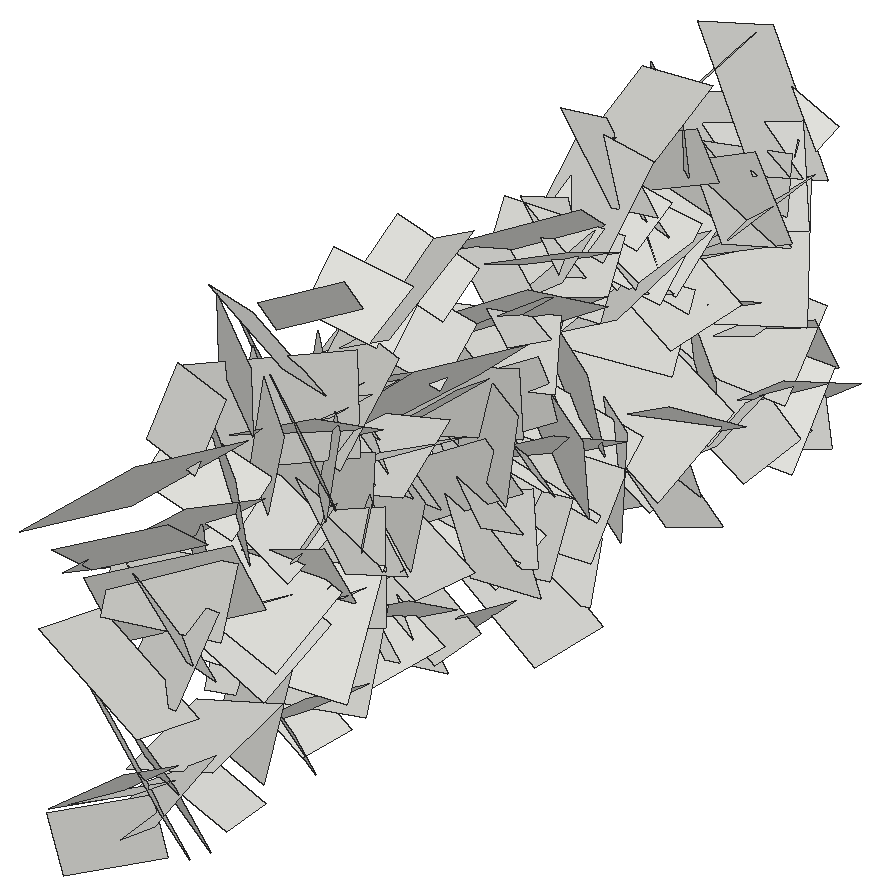
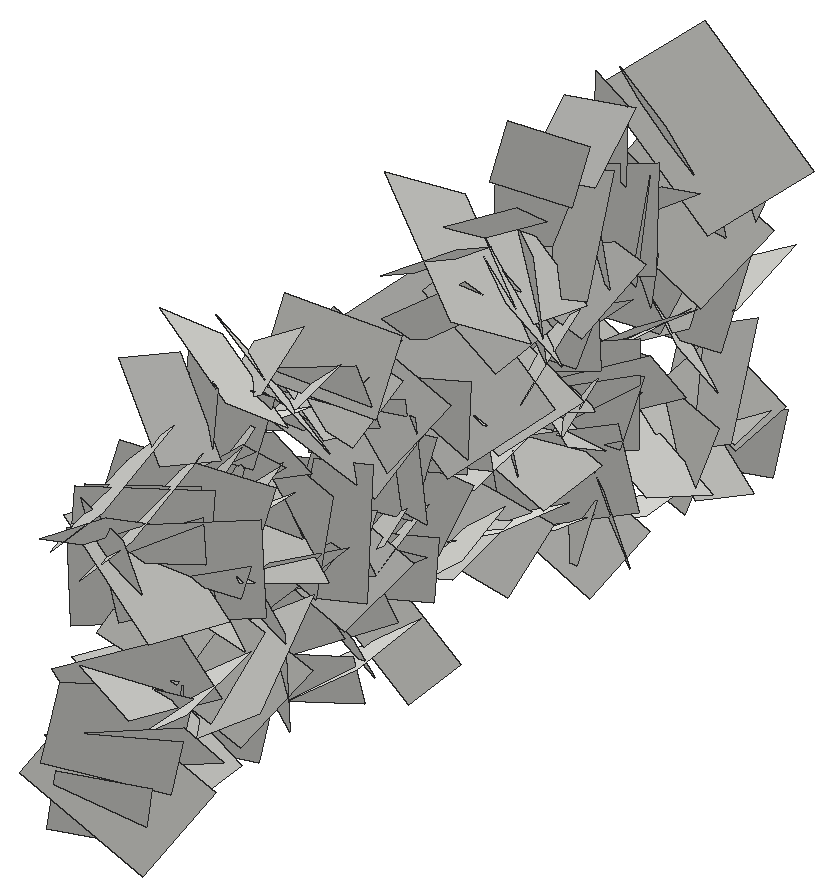
# SketchUp Ruby script. Lengths in inches.
U = 1.inch
M = Sketchup.active_model
def pt(a) = Geom::Point3d.new(a.map { |v| v * U })
def face(e, loops, mat)
  f = e.add_face(loops[0].map { |a| pt(a) })
  loops[1..].each { |l| e.add_face(l.map { |a| pt(a) }).erase! }
  f.material = f.back_material = mat if mat
  f
end
# faces: each face lists its corners as indices into pts; further lists are holes
def faces(e, pts, list, mat = nil) = list.each { |f| face(e, (f[0].is_a?(Array) ? f : [f]).map { |l| l.map { |i| pts[i] } }, mat) }
# xy, xz, yz: faces in a plane at the given z, y or x. An outline is a flat list of corners, or four numbers for a rectangle; further outlines are holes
def ring(l) = l.size == 4 ? [[l[0], l[1]], [l[2], l[1]], [l[2], l[3]], [l[0], l[3]]] : l.each_slice(2).to_a
def flat(e, list, mat, &to3) = list.each { |f| face(e, (f[0].is_a?(Array) ? f : [f]).map { |l| ring(l).map { |u, v| to3.(u, v) } }, mat) }
def xy(e, z, list, mat = nil) = flat(e, list, mat) { |x, y| [x, y, z] }
def xz(e, y, list, mat = nil) = flat(e, list, mat) { |x, z| [x, y, z] }
def yz(e, x, list, mat = nil) = flat(e, list, mat) { |y, z| [x, y, z] }
def lines(e, pts, list) = list.each { |a, b| e.add_line(pt(pts[a]), pt(pts[b])) }
# prism: a flat outline (further loops are holes) pulled along v
def prism(e, loops, v, mat = nil)
  f = face(e, loops, mat); d = Geom::Vector3d.new(v.map { |x| x * U })
  f.pushpull(f.normal.samedirection?(d) ? d.length : -d.length)
end
def box(e, o, s, mat = nil) = prism(e, [[o, [o[0] + s[0], o[1], o[2]], [o[0] + s[0], o[1] + s[1], o[2]], [o[0], o[1] + s[1], o[2]]]], [0, 0, s[2]], mat)
def at(x, y, z, deg = 0) = Geom::Transformation.translation(pt([x, y, z])) * Geom::Transformation.rotation(ORIGIN, Z_AXIS, deg.degrees)
def axes(o, x, y, z) = Geom::Transformation.new([*x, 0, *y, 0, *z, 0, *pt(o).to_a, 1])
def part(name) = M.definitions.add(name)
# library, detail: a bought-in or finely detailed component or shape, given as its bounding box
def library(name, o, s) = part(name).tap { |d| box(d.entities, o, s) }
def detail(e, o, s) = box(e.add_group.entities, o, s)
def put(e, d, t, mat = nil) = e.add_instance(d, t).tap { |i| i.material = mat if mat }
def group(e, t, mat = nil) = e.add_group.tap { |g| g.transformation = t; g.material = mat if mat }.entities
root = M.entities
c1 = part("Component\#6")
p = [[0.01,0,0],[0,3.24,4.54],[4.32,3.24,4.54],[4.33,0,0]]
faces(c1.entities,p,[[0,1,2,3]])
put(root,c1,axes([400.91,170.73,19.61],[-0.06378,-0.15247,0.68566],[-0.07422,0.68605,0.14641],[0.74085,0.05561,0.0737]))
put(root,c1,axes([400.91,173.11,21.9],[-0.05319,-0.68826,0.19248],[-0.04456,0.19546,0.68797],[0.75624,-0.03689,0.05408]))
put(root,c1,axes([400.91,173.15,22.23],[0.01199,-0.5915,0.12784],[0.10227,0.12799,0.58366],[0.63327,-0.00947,-0.09668]))
put(root,c1,axes([404.88,174.01,26.46],[0.07872,-0.97306,0.24072],[-0.0738,0.23579,0.97461],[-1.05998,-0.08868,-0.04998]))
put(root,c1,axes([404.88,172.13,35.78],[-0.07615,0.65901,-0.5201],[-0.04859,-0.52431,-0.658],[-0.88857,-0.02781,0.08055]))
put(root,c1,axes([404.88,173.5,20.5],[0.29119,-0.77592,0.90535],[-0.00734,0.92801,0.79744],[-1.26387,-0.18415,0.20396]))
put(root,c1,axes([404.88,170.16,39.2],[0.24703,1.2789,-0.21613],[0.13589,-0.24123,-1.28918],[-1.36812,0.20696,-0.16707]))
put(root,c1,axes([404.88,171.36,22.89],[-0.02535,0.88672,0.32576],[0.06435,0.32663,-0.88464],[-0.99927,-0.00146,-0.06523]))
put(root,c1,axes([404.88,173.31,35.98],[0.01252,1.07454,-0.37217],[0.12805,-0.37127,-1.06811],[-1.19858,-0.02844,-0.11799]))
put(root,c1,axes([404.88,176.41,32.2],[-0.11408,-0.0942,-0.79779],[-0.0272,-0.8041,0.09841],[-0.85109,0.03832,0.10379]))
put(root,c1,axes([404.88,172.625,27.43],[0.01975,0.58315,0.74345],[-0.01761,0.74368,-0.58292],[-1.00141,-0.00157,0.02491]))
put(root,c1,axes([404.88,174.78,20.26],[-0.10048,-0.39109,0.79293],[-0.10042,0.79738,0.38196],[-0.93179,-0.04376,-0.12667]))
put(root,c1,axes([400.91,174.375,32.02],[-0.18574,0.64681,-0.5499],[-0.00393,-0.56207,-0.65994],[0.8999,0.13105,-0.11638]))
put(root,c1,axes([404.88,176.05,33.17],[-0.01986,0.50916,-0.88553],[0.06176,-0.8837,-0.50934],[-1.08099,-0.05984,-0.01283]))
put(root,c1,axes([400.91,177.7,39.03],[-0.08239,-0.33737,-0.64844],[0.10668,-0.65083,0.32654],[0.76743,0.05425,-0.11501]))
put(root,c1,axes([400.91,178.15,33.23],[0.08938,-0.00525,-0.60269],[-0.06829,-0.60515,-0.00374],[0.63521,-0.06432,0.0844]))
put(root,c1,axes([404.88,174.9,23.69],[0.06803,0.90477,0.33383],[-0.16872,0.33992,-0.89067],[-1.00823,0.00417,0.17157]))
put(root,c1,axes([400.91,175.43,34.87],[-0.0411,0.62613,0.35799],[-0.03637,0.3565,-0.62724],[0.76365,0.05068,-0.01061]))
put(root,c1,axes([400.91,176.44,21.6],[-0.04345,0.60879,-0.00304],[0.10651,0.00376,-0.60183],[0.63647,0.04093,0.10051]))
put(root,c1,axes([404.88,177.13,31.79],[0.078,-0.30439,1.03044],[0.07955,1.03178,0.29943],[-1.13614,0.05135,0.09171]))
put(root,c1,axes([404.88,182.1,27.04],[0.18817,-1.1788,-0.21223],[0.10509,-0.19936,1.19019],[-1.26526,-0.19187,0.06729]))
put(root,c1,axes([400.91,180.11,41],[-0.0874,0.13713,-0.78202],[-0.02965,-0.78624,-0.13492],[0.84107,-0.01347,-0.08602]))
put(root,c1,axes([400.91,180.68,27.18],[-0.06604,-0.60003,0.10008],[0.10227,0.08959,0.59716],[0.63666,-0.07663,-0.08554]))
put(root,c1,axes([404.88,182.77,28.15],[0.11013,-1.0722,-0.31704],[0.03816,-0.31503,1.07721],[-1.18456,-0.10983,0.00522]))
put(root,c1,axes([404.88,178.01,21.81],[-0.00864,0.40014,0.99077],[0.02339,0.99065,-0.39991],[-1.13239,0.01741,-0.01582]))
put(root,c1,axes([400.91,182.27,37.76],[-0.22679,0.05489,-0.89691],[-0.06736,-0.9206,-0.04118],[0.95012,-0.05216,-0.217]))
put(root,c1,axes([404.88,181.8125,37.17],[0.0246,-0.63961,0.56311],[-0.17949,0.54862,0.63013],[-0.88529,-0.129,-0.11211]))
put(root,c1,axes([404.88,185.38,28.27],[0.28552,-0.8956,-0.93898],[0.07116,-0.9481,0.92355],[-1.37362,-0.23528,-0.14733]))
put(root,c1,axes([404.88,183.67,38.38],[-0.04708,0.10578,-1.15378],[0.2342,-1.13267,-0.11235],[-1.2056,-0.22416,0.02323]))
put(root,c1,axes([400.91,179.78,31.84],[-0.01485,0.68647,0.23212],[-0.1576,0.2245,-0.67291],[0.75179,0.06062,-0.13648]))
put(root,c1,axes([404.88,181.64,30.57],[-0.02444,0.48831,-0.77146],[-0.19424,-0.75848,-0.47462],[-0.9481,0.1428,0.11713]))
put(root,c1,axes([400.91,183.98,26.9],[-0.15473,-0.64925,-0.29626],[0.07231,-0.3137,0.65387],[0.75301,-0.10329,-0.12366]))
put(root,c1,axes([400.91,181.88,29.24],[0.0732,0.47057,-0.46808],[-0.06498,-0.46407,-0.47558],[0.70054,-0.09222,0.00479]))
put(root,c1,axes([404.88,180.55,24.45],[-0.04702,0.95483,-0.28451],[0.08229,-0.28062,-0.95386],[-1.05288,-0.06457,-0.06184]))
put(root,c1,axes([400.91,182.11,23.57],[-0.01533,0.32032,-0.55846],[0.07998,-0.55391,-0.31966],[0.67773,0.07262,0.02509]))
put(root,c1,axes([404.88,182.41,31.86],[0.21699,-0.67676,1.03332],[-0.0082,1.04669,0.68705],[-1.3093,-0.11872,0.16695]))
put(root,c1,axes([404.88,181.12,36.49],[0.0887,0.85058,-0.45713],[-0.14057,-0.44437,-0.85112],[-1.01388,0.13603,0.07801]))
put(root,c1,axes([400.91,184.65,28.76],[0.04824,-0.62434,-0.28052],[-0.09786,-0.28417,0.61748],[0.7189,0.00321,0.10288]))
put(root,c1,axes([404.88,185.4,30.76],[0.02152,-0.00963,-1.2106],[0.23963,-1.18945,0.01326],[-1.26071,-0.22625,-0.01814]))
put(root,c1,axes([400.91,181.75,22.9],[0.07496,0.59984,0.04506],[0.05269,0.03939,-0.60235],[0.63545,-0.07402,0.04463]))
put(root,c1,axes([404.88,185.55,26.35],[-0.05433,-0.24183,-1.04679],[0.06418,-1.04696,0.23891],[-1.13701,-0.04754,0.0635]))
put(root,c1,axes([404.88,184.8,33.37],[-0.19651,0.19461,-0.78555],[0.01158,-0.80522,-0.20206],[-0.85778,-0.05545,0.17724]))
put(root,c1,axes([400.91,183.74,37.84],[0.08456,-0.37494,0.46177],[-0.03825,0.46199,0.38136],[0.62935,0.07846,-0.03886]))
put(root,c1,axes([400.91,183.4375,30.23],[-0.10865,-0.24445,0.66529],[0.00738,0.67183,0.24793],[0.75127,-0.04195,0.09378]))
put(root,c1,axes([400.91,186.27,36.66],[-0.23271,0.08267,-1.0169],[-0.17131,-1.02986,-0.04883],[1.06781,-0.14721,-0.22945]))
put(root,c1,axes([404.88,182.86,27.86],[-0.00866,0.87216,-0.09866],[-0.12421,-0.09886,-0.86427],[-0.92206,0.00513,0.11735]))
put(root,c1,axes([400.91,186.9,33.68],[-0.12726,-0.80704,-0.07778],[0.05104,-0.08559,0.81372],[0.85791,-0.11462,-0.05995]))
put(root,c1,axes([404.88,186.8,27.07],[0.11611,-1.02809,0.5245],[0.14127,0.5346,1.02006],[-1.21522,-0.03608,0.16869]))
put(root,c1,axes([404.88,182.62,33.52],[0.16113,0.63843,0.91206],[0.00988,0.91976,-0.64538],[-1.18006,0.09488,0.11913]))
put(root,c1,axes([400.91,188.3,31.13],[-0.1103,-0.11339,-0.88165],[-0.13763,-0.87621,0.12802],[0.93214,-0.14279,-0.08543]))
put(root,c1,axes([400.91,188.62,32.29],[-0.0866,-0.74743,0.19758],[-0.06186,0.20408,0.74787],[0.81715,-0.06376,0.07755]))
put(root,c1,axes([400.91,185.35,37.93],[-0.06077,0.5182,0.40006],[0.00909,0.40215,-0.51968],[0.69387,0.04012,0.04185]))
put(root,c1,axes([404.88,189.07,22.99],[-0.09993,-0.91741,-0.05408],[-0.10319,-0.04408,0.91762],[-0.96866,0.09934,-0.09218]))
put(root,c1,axes([404.88,184.85,32.98],[0.15473,1.07562,-0.16592],[-0.16403,-0.14519,-1.07739],[-1.14193,0.1666,0.13228]))
put(root,c1,axes([404.88,186.85,26],[-0.04759,0.74401,-0.43208],[-0.09551,-0.43435,-0.73856],[-0.90698,0.0067,0.10045]))
put(root,c1,axes([404.88,186.48,30.64],[-0.03295,0.70699,0.47041],[-0.18441,0.45544,-0.69599],[-0.88105,-0.12176,0.12808]))
put(root,c1,axes([400.91,189.49,31],[-0.19159,0.03614,-0.77666],[0.1449,-0.78347,-0.06827],[0.81131,0.14846,-0.17121]))
put(root,c1,axes([404.88,189.24,21.76],[-0.15995,-0.688,0.38857],[0.02017,0.39231,0.70202],[-0.83731,0.14088,-0.05731]))
put(root,c1,axes([404.88,190.89,25.45],[0.07637,-0.93381,0.1535],[-0.06656,0.14888,0.93522],[-1.00091,-0.08115,-0.05048]))
put(root,c1,axes([400.91,188.48,31.6],[0.00806,0.51701,-0.38199],[0.06142,-0.38101,-0.51453],[0.67861,0.02834,0.0511]))
put(root,c1,axes([404.88,185.63,37.94],[0.10296,1.07287,0.66666],[0.13207,0.65722,-1.07584],[-1.33238,0.14805,-0.05512]))
put(root,c1,axes([404.88,187.18,35.87],[0.21905,1.32848,-0.23139],[0.18572,-0.25856,-1.32798],[-1.41727,0.17144,-0.20979]))
put(root,c1,axes([400.91,188.01,25.87],[-0.18323,0.88768,-0.1275],[-0.06793,-0.14175,-0.89995],[0.94816,0.16139,-0.08912]))
put(root,c1,axes([400.91,188.41,35.3125],[0.03073,0.48255,0.4704],[-0.10717,0.46862,-0.47449],[0.70624,0.05011,-0.09248]))
put(root,c1,axes([400.91,188.93,38.32],[-0.06934,0.59373,0.25],[0.00198,0.25145,-0.59671],[0.68287,0.05956,0.02711]))
put(root,c1,axes([400.91,193.29,29.97],[0.02765,-0.60791,0.13872],[-0.08921,0.13414,0.60366],[0.6549,0.04394,0.07638]))
put(root,c1,axes([400.91,192.39,25.48],[-0.15082,-0.34829,0.66058],[-0.01541,0.67363,0.35204],[0.79143,-0.05326,0.13274]))
put(root,c1,axes([404.88,193.58,33.2],[-0.1306,0.22319,-0.86205],[-0.05382,-0.87061,-0.21815],[-0.94237,0.01879,0.13193]))
put(root,c1,axes([400.91,194.26,19.42],[-0.05867,-0.70774,0.13488],[-0.12622,0.14241,0.69835],[0.75321,-0.03127,0.12754]))
put(root,c1,axes([404.88,192.76,27.5],[0.21382,-0.08753,1.03604],[-0.20559,1.03367,0.1251],[-1.08277,-0.21355,0.18084]))
put(root,c1,axes([400.91,192.62,23.41],[-0.0945,0.05137,0.75973],[0.00531,0.76494,-0.05113],[0.80713,0.00098,0.08928]))
put(root,c1,axes([400.91,193.25,29.42],[-0.0602,0.67546,-0.3863],[-0.10598,-0.39045,-0.66802],[0.81797,-0.00088,-0.11498]))
put(root,c1,axes([404.88,194.92,22.54],[-0.07164,-0.895,0.57486],[0.24411,0.55005,0.88344],[-1.1008,0.18023,0.15849]))
put(root,c1,axes([400.91,192.68,25.51],[0.10584,0.56729,0.32604],[-0.07365,0.33715,-0.56532],[0.68964,-0.05105,-0.11041]))
put(root,c1,axes([400.91,194.0625,27.88],[-0.03826,-0.32146,0.75655],[-0.14724,0.74878,0.31153],[0.85881,0.11405,0.08712]))
put(root,c1,axes([400.91,194.1,30.97],[-0.07757,0.18705,0.69229],[0.05179,0.69557,-0.18277],[0.75837,-0.02837,0.08329]))
put(root,c1,axes([404.88,194.12,36.42],[0.16155,0.92195,-0.51802],[-0.06641,-0.51458,-0.93426],[-1.119,0.16364,-0.01934]))
put(root,c1,axes([400.91,194.71,36.49],[-0.01491,0.71707,-0.22931],[-0.11795,-0.22881,-0.70868],[0.78925,-0.02064,-0.11024]))
put(root,c1,axes([404.88,195.125,35.61],[-0.03117,0.92717,-0.40656],[0.02653,-0.40594,-0.92757],[-1.07281,-0.03698,-0.01113]))
put(root,c1,axes([404.88,198.72,19.65],[0.06387,-1.04135,0.05905],[0.06023,0.06234,1.04135],[-1.10396,-0.05685,0.06023]))
put(root,c1,axes([400.91,196.3,29.33],[-0.09147,0.43894,-0.4809],[0.05464,-0.47898,-0.44644],[0.688,0.09639,-0.02848]))
put(root,c1,axes([404.88,195.45,23.05],[-0.08121,0.42866,0.62692],[-0.16296,0.6083,-0.43472],[-0.78836,-0.1699,0.02528]))
put(root,c1,axes([404.88,195.7,29.31],[0.12944,0.87645,-0.3909],[-0.13192,-0.37627,-0.88251],[-1.00866,0.16168,0.06525]))
put(root,c1,axes([404.88,197.34,38.49],[-0.22162,0.66132,-0.53694],[0.02723,-0.54773,-0.68462],[-0.90256,-0.17891,0.1112]))
put(root,c1,axes([404.88,196.41,37.05],[-0.02372,0.78814,-0.36288],[-0.15491,-0.36124,-0.77556],[-0.90659,0.0411,0.14202]))
put(root,c1,axes([404.88,200.17,25.9],[-0.12286,-0.34825,-0.84521],[0.12526,-0.85054,0.33424],[-0.96086,-0.06635,0.15165]))
put(root,c1,axes([404.88,197.85,24.73],[0.35143,-0.52734,1.13432],[-0.18025,1.14359,0.58135],[-1.31365,-0.29799,0.22369]))
put(root,c1,axes([400.91,199.74,34.07],[0.11183,-0.60219,-0.2199],[-0.02555,-0.22643,0.6085],[0.67907,0.09065,0.0591]))
put(root,c1,axes([400.91,197.11,20.7],[-0.0234,0.20043,0.60552],[0.11848,0.59772,-0.19378],[0.66563,-0.09934,0.05578]))
put(root,c1,axes([404.88,200.08,36.17],[-0.04967,-0.3024,-0.77978],[-0.15753,-0.76557,0.30582],[-0.87244,0.15545,-0.01082]))
put(root,c1,axes([400.91,196.5,26.6],[-0.00001,0.64808,0.59207],[-0.20568,0.57742,-0.63205],[0.90746,0.13088,-0.14325]))
put(root,c1,axes([400.91,198.68,37.125],[0.06347,0.58127,-0.24952],[-0.07215,-0.24326,-0.58302],[0.66662,-0.08167,-0.03935]))
put(root,c1,axes([404.88,198.8,27.02],[0.0226,-0.2767,0.96977],[-0.06915,0.96758,0.27751],[-1.06674,-0.06859,0.00256]))
put(root,c1,axes([404.88,198.67,35.61],[0.10111,0.59855,0.78971],[-0.15679,0.79307,-0.58323],[-1.03859,-0.06146,0.16492]))
put(root,c1,axes([404.88,199.8,22.82],[0.00598,0.07204,1.08492],[0.02761,1.08461,-0.07215],[-1.15221,0.02636,0.0039]))
put(root,c1,axes([400.91,201.07,39.9375],[-0.03161,0.68058,-0.41337],[-0.06223,-0.41441,-0.67806],[0.84176,-0.00508,-0.06565]))
put(root,c1,axes([400.91,200.57,36.04],[-0.10099,0.61602,0.17436],[0.1325,0.19079,-0.60575],[0.66557,0.05549,0.14705]))
put(root,c1,axes([404.88,206.72,25.52],[0.07134,-1.27871,-0.42932],[0.37284,-0.39835,1.24159],[-1.38032,-0.17369,0.31318]))
put(root,c1,axes([404.88,204.74,34.65],[-0.08046,-0.48471,-0.63269],[-0.12911,-0.62103,0.49039],[-0.83492,0.14274,-0.01486]))
put(root,c1,axes([400.91,200.85,29.625],[-0.04324,0.39016,0.69087],[-0.10275,0.68414,-0.39209],[0.83473,0.10443,-0.01247]))
put(root,c1,axes([404.88,199.54,32.72],[0.14681,1.15124,0.44909],[0.05729,0.44582,-1.15954],[-1.30862,0.14867,-0.00039]))
put(root,c1,axes([400.91,202.42,34.22],[-0.03507,0.56649,-0.26791],[0.06705,-0.26389,-0.56581],[0.66085,0.05684,0.04319]))
put(root,c1,axes([404.88,206.07,20.81],[0.31441,-1.20333,0.63493],[0.01893,0.65323,1.22967],[-1.44208,-0.25378,0.15457]))
put(root,c1,axes([404.88,201.41,38.375],[0.12316,0.77538,0.57304],[-0.12545,0.58429,-0.76661],[-1.01427,0.02189,0.1644]))
put(root,c1,axes([400.91,204.22,36.67],[0.08595,0.41822,-0.43473],[-0.01861,-0.43682,-0.42351],[0.63917,-0.06896,0.04613]))
put(root,c1,axes([400.91,204.95,35.05],[0.03568,0.1968,-0.61743],[-0.04358,-0.61637,-0.1987],[0.68554,-0.04943,0.01951]))
put(root,c1,axes([404.88,202.75,27.49],[0.17368,0.85862,-0.51485],[-0.1903,-0.48804,-0.87105],[-1.04401,0.2318,0.07312]))
put(root,c1,axes([400.91,203.96,20.97],[0.02025,-0.24988,0.58047],[-0.03388,0.57961,0.25056],[0.66903,0.03691,-0.00488]))
put(root,c1,axes([400.91,202.23,33.91],[0.02493,0.60398,0.49928],[-0.17768,0.49182,-0.58706],[0.81142,0.08914,-0.14389]))
put(root,c1,axes([400.91,204.33,34.72],[-0.02793,-0.28222,0.66343],[0.05268,0.66158,0.28341],[0.7624,-0.05605,0.00473]))
put(root,c1,axes([404.88,207.21,30.03],[0.00943,-1.01637,-0.0193],[0.00822,-0.01923,1.01638],[-1.07752,-0.00904,0.00758]))
put(root,c1,axes([400.91,207.84,29.22],[-0.13906,-0.51177,-0.49755],[0.00544,-0.50655,0.51967],[0.75658,-0.09042,-0.09518]))
put(root,c1,axes([400.91,206.625,39.5],[-0.00312,0.09172,-0.66161],[0.00201,-0.66161,-0.09173],[0.70801,0.00228,-0.00265]))
put(root,c1,axes([404.88,208.01,36.375],[0.10923,0.38133,-1.06486],[-0.05778,-1.06635,-0.38714],[-1.19755,0.08623,-0.07845]))
put(root,c1,axes([404.88,205.67,24.52],[-0.15369,0.87531,0.08009],[0.01982,0.08422,-0.88666],[-0.9315,-0.14262,-0.03208]))
put(root,c1,axes([400.91,208.95,27.68],[-0.1117,0.11156,-0.75397],[-0.06454,-0.75994,-0.10393],[0.80532,-0.04543,-0.11291]))
put(root,c1,axes([400.91,210.37,37.54],[-0.0852,-0.7988,-0.26142],[-0.21653,-0.23617,0.78446],[0.8642,-0.13792,0.17078]))
put(root,c1,axes([404.88,211.43,33.78],[0.23599,-0.36182,-1.29322],[0.09706,-1.30373,0.38052],[-1.42014,-0.14923,-0.18889]))
put(root,c1,axes([400.91,206.77,29.69],[0.13468,0.0618,0.68245],[-0.14259,0.68282,-0.03679],[0.71222,0.12502,-0.13642]))
put(root,c1,axes([400.91,209.27,26.93],[0.01951,-0.6006,0.29742],[0.06663,0.29777,0.59742],[0.70729,-0.01148,-0.06448]))
put(root,c1,axes([404.88,211.47,22.62],[0.20513,-1.22241,0.07319],[0.04122,0.08019,1.23659],[-1.29742,-0.19072,0.05085]))
put(root,c1,axes([404.88,210.23,35.31],[-0.06568,0.00099,-0.81141],[-0.08224,-0.81005,0.00494],[-0.85616,0.07773,0.06177]))
put(root,c1,axes([404.88,206.36,33.23],[0.09168,1.1059,0.20164],[0.04784,0.19866,-1.1089],[-1.19063,0.09314,-0.02903]))
put(root,c1,axes([400.91,207.11,31.75],[-0.23783,0.22127,0.93353],[-0.03566,0.95632,-0.23476],[1.01634,0.08533,0.21022]))
put(root,c1,axes([404.88,210.61,30.96],[-0.02538,-1.03384,0.49264],[0.2847,0.47394,1.00764],[-1.18007,0.13657,0.23251]))
put(root,c1,axes([404.88,212.41,27.7],[-0.11035,-0.46639,-0.85158],[0.0233,-0.85737,0.46687],[-1.02892,0.03061,0.1019]))
put(root,c1,axes([404.88,212.85,24.81],[0.10314,-0.72888,-0.73382],[-0.20394,-0.73695,0.70648],[-1.07722,0.06973,-0.20401]))
put(root,c1,axes([400.91,212.36,26.625],[-0.06935,-0.64087,-0.11796],[0.11905,-0.12787,0.63241],[0.68039,-0.04294,-0.12268]))
put(root,c1,axes([404.88,209.77,25.57],[0.04769,1.02209,-0.46416],[0.05126,-0.46587,-1.02116],[-1.18879,0.02092,-0.06265]))
put(root,c1,axes([404.88,212.48,33.12],[-0.02538,-1.03384,0.49264],[0.2847,0.47394,1.00764],[-1.18007,0.13657,0.23251]))
put(root,c1,axes([404.88,211.63,27.44],[-0.13698,0.50835,-0.7639],[-0.02564,-0.77306,-0.51036],[-0.97231,-0.05123,0.12108]))
put(root,c1,axes([400.91,212.78,35.18],[-0.06835,-0.19577,-0.64021],[0.13077,-0.63563,0.18195],[0.69749,0.09999,-0.09685]))
put(root,c1,axes([400.91,211.4,20.36],[-0.11841,0.02386,0.67628],[0.07272,0.6823,-0.01274],[0.7136,-0.06557,0.11352]))
put(root,c1,axes([400.91,211.1,35.2],[0.07899,0.5337,0.27791],[0.02897,0.27674,-0.53878],[0.63716,-0.07875,-0.00996]))
